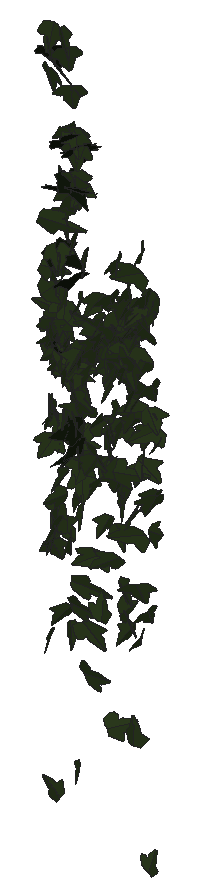
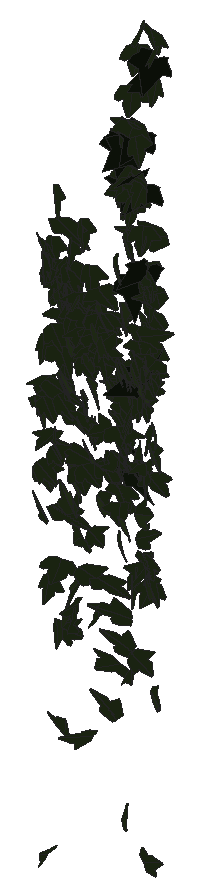
# SketchUp Ruby script. Lengths in millimetres.
U = 1.mm
M = Sketchup.active_model
def pt(a) = Geom::Point3d.new(a.map { |v| v * U })
def face(e, loops, mat)
  f = e.add_face(loops[0].map { |a| pt(a) })
  loops[1..].each { |l| e.add_face(l.map { |a| pt(a) }).erase! }
  f.material = f.back_material = mat if mat
  f
end
# faces: each face lists its corners as indices into pts; further lists are holes
def faces(e, pts, list, mat = nil) = list.each { |f| face(e, (f[0].is_a?(Array) ? f : [f]).map { |l| l.map { |i| pts[i] } }, mat) }
# xy, xz, yz: faces in a plane at the given z, y or x. An outline is a flat list of corners, or four numbers for a rectangle; further outlines are holes
def ring(l) = l.size == 4 ? [[l[0], l[1]], [l[2], l[1]], [l[2], l[3]], [l[0], l[3]]] : l.each_slice(2).to_a
def flat(e, list, mat, &to3) = list.each { |f| face(e, (f[0].is_a?(Array) ? f : [f]).map { |l| ring(l).map { |u, v| to3.(u, v) } }, mat) }
def xy(e, z, list, mat = nil) = flat(e, list, mat) { |x, y| [x, y, z] }
def xz(e, y, list, mat = nil) = flat(e, list, mat) { |x, z| [x, y, z] }
def yz(e, x, list, mat = nil) = flat(e, list, mat) { |y, z| [x, y, z] }
def lines(e, pts, list) = list.each { |a, b| e.add_line(pt(pts[a]), pt(pts[b])) }
# prism: a flat outline (further loops are holes) pulled along v
def prism(e, loops, v, mat = nil)
  f = face(e, loops, mat); d = Geom::Vector3d.new(v.map { |x| x * U })
  f.pushpull(f.normal.samedirection?(d) ? d.length : -d.length)
end
def box(e, o, s, mat = nil) = prism(e, [[o, [o[0] + s[0], o[1], o[2]], [o[0] + s[0], o[1] + s[1], o[2]], [o[0], o[1] + s[1], o[2]]]], [0, 0, s[2]], mat)
def at(x, y, z, deg = 0) = Geom::Transformation.translation(pt([x, y, z])) * Geom::Transformation.rotation(ORIGIN, Z_AXIS, deg.degrees)
def axes(o, x, y, z) = Geom::Transformation.new([*x, 0, *y, 0, *z, 0, *pt(o).to_a, 1])
def part(name) = M.definitions.add(name)
# library, detail: a bought-in or finely detailed component or shape, given as its bounding box
def library(name, o, s) = part(name).tap { |d| box(d.entities, o, s) }
def detail(e, o, s) = box(e.add_group.entities, o, s)
def put(e, d, t, mat = nil) = e.add_instance(d, t).tap { |i| i.material = mat if mat }
def group(e, t, mat = nil) = e.add_group.tap { |g| g.transformation = t; g.material = mat if mat }.entities
root = M.entities
M.materials.add("efeu1").color = [18, 25, 13]
M.materials.add("efeu2").color = [43, 57, 29]
c1 = part("ivyleaf_10")
p = [[0,12.8,-0.8],[-1.5,51.3,-10.9],[-4.9,51,-11.6],[-13.6,26.5,-7.3],[-13.2,15.9,-4.6],[-21.1,19.3,-7.2],
  [-29.5,16.3,-8.3],[-29.2,8.3,-6.2],[-19.7,-9.8,0.5],[-7.6,-13,4],[1,-12.2,5.8],[-0.4,51.1,-11.1],
  [-1.5,51.1,-10.9],[1,-12.4,5.9],[16.9,-12.4,3.5],[35.1,9.1,-5.1],[35,12.9,-6.1],[20.5,16.4,-4.9],
  [15.8,15,-3.8],[15.3,27.6,-7.1],[12.8,31.3,-7.8]]
faces(c1.entities,p,[[0,1,2,3,4,5,6,7,8,9,10],[11,12,0,13,14,15,16,17,18,19,20]],"efeu2")
c2 = part("ivyleaf_9")
p = [[39.1,54.8,31.7],[34.5,51.8,30.2],[-5.3,25.2,17.3],[-17.9,28.3,20.9],[-21.6,21.7,17],[-20.2,4.3,5.3],
  [-22.9,-0.3,2.5],[-17.1,-4,-0.6],[-2,-2.1,-1.2],[-0.7,-15.4,-10.1],[16.6,-22.3,-16.7],[21.1,-15.1,-12.5],
  [32.7,-10.7,-11],[46.1,-1.8,-6.6],[30.8,11.2,3.8]]
faces(c2.entities,p,[[0,1,2,3,4,5,6,7,8,9,10,11,12,13,14]],"efeu1")
put(root,c1,axes([788.1,1030.8,1427.8],[-0.8216,0.31601,0.08048],[-0.10582,0.00442,-0.74318],[-0.38351,-0.67822,0.03266]))
put(root,c1,axes([783.8,1037.2,366.4],[0.35503,-0.51907,0.28916],[0.17558,-0.25081,-0.59507],[0.70331,0.32464,0.00259]))
put(root,c1,axes([799.3,1035.4,70.7],[0.41211,-0.03589,0.60831],[-0.74004,0.04654,0.33959],[-0.07091,-0.69425,-0.00868]))
put(root,c1,axes([791.1,1037.6,927.4],[-0.31775,-0.66613,-0.05139],[0.00589,0.0522,-0.68667],[1.27154,-0.1667,-0.00966]))
put(root,c1,axes([800.6,1033.4,982.4],[0.2874,0.16747,0.66778],[-0.64392,-0.40925,0.28883],[0.5393,-0.57788,-0.01102]))
put(root,c2,axes([787.2,1031.5,1468.6],[0.6978,0.49681,-0.19291],[-0.15856,-0.14442,-0.75725],[-0.63057,0.58609,-0.02307]))
put(root,c1,axes([791.7,1032.9,898],[0.77102,0.08245,0.22157],[-0.26965,-0.01835,0.63726],[0.10235,-0.66944,0.00982]))
put(root,c1,axes([778.7,1041.7,950.2],[0.68596,0.18794,0.34559],[0.39955,0.11033,-0.59284],[-0.26587,0.65069,0.00071]))
put(root,c1,axes([799.9,1015.8,799.9],[0.1243,-0.11012,0.73702],[-0.66756,0.49393,0.14944],[-0.61718,-0.55643,-0.0132]))
put(root,c1,axes([792.3,1029.1,785.9],[0.2141,-0.65009,-0.01518],[0.00013,0.01541,-0.65975],[1.23759,0.11246,0.00269]))
put(root,c1,axes([793.1,1027.7,737.6],[0.73244,0.27951,-0.31616],[-0.34633,-0.13931,-0.66221],[-0.38094,0.66407,-0.00585]))
put(root,c1,axes([788.2,1029.7,1483.2],[-0.28744,0.74297,-0.0561],[0.00406,-0.05779,-0.7793],[-0.909,-0.2352,0.01426]))
put(root,c1,axes([797.4,1029.2,926.8],[0.31491,-0.02662,0.66088],[-0.48842,0.55843,0.17886],[-0.64233,-0.43767,0.18801]))
put(root,c1,axes([793.6,1033.7,556],[0.21115,-0.73707,0.09646],[-0.00653,-0.10027,-0.75661],[0.90687,0.17089,-0.02791]))
put(root,c1,axes([792.8,1042.4,897.2],[-0.01529,0.02833,0.67814],[0.09057,-0.67413,0.02954],[0.82309,0.07471,0.00935]))
put(root,c1,axes([793.5,1044.9,604.9],[0.83447,-0.2207,-0.05303],[-0.05883,0.02324,-0.71868],[0.27059,0.68565,0.00729]))
put(root,c1,axes([780.6,1028.3,1011.1],[0.68309,-0.13537,-0.48508],[0.56698,-0.14057,0.57566],[-0.2367,-0.72735,-0.02098]))
put(root,c1,axes([797.1,1043.7,878.8],[-0.07619,-0.6591,-0.00693],[0.00134,0.00686,-0.66205],[0.80415,-0.06246,0.00045]))
put(root,c1,axes([794.2,1036.8,564.8],[0.47786,-0.63117,0.09926],[0.07896,-0.07664,-0.74269],[0.77548,0.39673,0.01446]))
put(root,c1,axes([799.2,1028.6,591.4],[-0.32506,0.49635,0.38567],[-0.27259,0.31674,-0.562],[-0.71677,-0.34556,0.03883]))
put(root,c1,axes([793.7,1045.7,768.5],[0.39639,0.56977,-0.20295],[-0.12608,-0.19187,-0.60663],[-1.1442,0.21853,-0.00346]))
put(root,c1,axes([792.2,1027.3,1511],[0.91653,-0.22701,0.09119],[0.10411,-0.03284,-0.78478],[0.27971,0.75606,-0.00671]))
put(root,c1,axes([783.4,1027.2,1061.1],[-0.1807,-0.20858,-0.64289],[0.74252,0.24504,-0.21972],[0.35857,-0.61253,0.13101]))
put(root,c2,axes([801.5,1036.1,912.9],[0.18122,-0.67532,0.32709],[-0.03577,0.32796,0.69043],[-0.91475,-0.14661,0.0378]))
put(root,c1,axes([798.6,1023.2,951.7],[-0.19091,0.66075,0.24701],[-0.20959,0.2097,-0.66978],[-0.83469,-0.20378,0.11169]))
put(root,c1,axes([798.3,1031.9,935.2],[0.07288,-0.62882,-0.29154],[0.11181,0.29388,-0.62614],[1.31439,0.00987,0.06943]))
put(root,c1,axes([808.1,1033.5,1069.4],[0.29042,-0.0913,-0.66321],[-0.45833,0.5644,-0.21254],[0.67603,0.42187,0.14082]))
put(root,c1,axes([804.1,1038.4,939.6],[0.34517,-0.6149,-0.26073],[-0.05992,0.262,-0.6398],[1.26972,0.17952,0.04068]))
put(root,c1,axes([798.6,1025.5,544.7],[-0.59363,-0.39577,-0.2622],[0.25431,0.15923,-0.62717],[0.52037,-0.5293,0.00739]))
put(root,c1,axes([803.6,1039.9,1166.3],[-0.57926,-0.51111,-0.06286],[0.0462,0.05062,-0.69758],[0.62655,-0.47626,-0.00668]))
put(root,c1,axes([803.7,1033,743.6],[0.44885,-0.47733,-0.38288],[-0.02835,0.40573,-0.515],[1.16425,0.1939,0.13507]))
put(root,c1,axes([801.6,1021.3,1048.5],[0.70382,-0.53867,-0.29794],[0.06531,0.36507,-0.61744],[1.16973,0.30373,0.21374]))
put(root,c1,axes([801.7,1024.1,960.1],[-0.89528,-0.26816,-0.13173],[0.17561,-0.01121,-0.77906],[0.3194,-0.74548,0.0591]))
put(root,c1,axes([806,1032.1,893],[-0.53685,0.56978,0.24643],[-0.25649,0.14743,-0.71629],[-0.7126,-0.48231,0.07216]))
put(root,c1,axes([805.1,1018.8,807.1],[-0.51279,0.56779,0.11249],[-0.09933,0.07964,-0.70621],[-0.69914,-0.42776,0.01783]))
put(root,c1,axes([806.4,1037.6,632.5],[-0.02983,-0.02156,0.66723],[-0.01438,-0.66756,-0.022],[0.81432,-0.01258,0.02405]))
put(root,c1,axes([805.3,1025.6,1084],[0.74042,-0.59205,-0.15393],[0.02348,0.18998,-0.69951],[1.16401,0.37276,0.11203]))
put(root,c1,axes([796.1,1041,881.8],[0.26766,-0.51968,-0.31436],[0.36513,-0.19834,0.53676],[-0.64477,-0.32805,0.17347]))
put(root,c1,axes([809.4,1031.6,585.8],[0.02991,0.54049,-0.53466],[-0.31756,-0.49664,-0.51399],[-0.87145,0.19953,0.16895]))
put(root,c1,axes([808.2,1043.6,792.7],[-0.25794,0.57627,-0.25871],[-0.14917,-0.2779,-0.57795],[-1.19293,-0.08985,0.12821]))
put(root,c1,axes([813.5,1034.4,875.5],[-0.75172,0.38055,0.21329],[-0.24032,0.08664,-0.72364],[-0.47488,-0.64625,0.02858]))
put(root,c1,axes([804.4,1025.5,1100.7],[0.53358,0.59441,0.03481],[0.02364,0.02896,-0.73798],[-0.72604,0.43779,0.00155]))
put(root,c1,axes([815.2,1040.2,422.2],[-0.2053,-0.57396,0.34459],[-0.10385,-0.34034,-0.58396],[1.26988,-0.12063,0.00795]))
put(root,c1,axes([811.7,1045,1320.9],[-0.14471,-0.72719,-0.02028],[0.01042,0.01915,-0.73678],[0.88745,-0.1188,0.00535]))
put(root,c2,axes([795.6,1037.4,1436.5],[0.77726,-0.42672,0.06495],[0.05255,-0.05237,-0.76655],[0.52396,0.63826,-0.01947]))
put(root,c1,axes([807.4,1040.3,968.4],[0.79768,0.23933,-0.04503],[-0.05019,-0.01861,-0.69625],[-0.29283,0.65512,-0.00333]))
put(root,c1,axes([810,1039.5,1237.5],[-0.75298,0.34973,-0.07002],[0.06708,-0.04498,-0.70929],[-0.42993,-0.61953,0.01197]))
put(root,c1,axes([805.1,1036.6,578.9],[0.34309,0.56152,0.42564],[0.12442,0.42103,-0.62281],[-0.85058,0.28808,0.08059]))
put(root,c1,axes([809.7,1038.4,672.6],[0.17239,-0.27183,0.6442],[0.33118,-0.62038,-0.28625],[1.28885,0.19577,-0.01261]))
put(root,c1,axes([812.4,1033.4,1018],[0.67283,-0.43188,0.01125],[0.01059,-0.00716,-0.70048],[0.52696,0.55157,-0.00028]))
put(root,c2,axes([804.3,1028.5,1101.2],[0.05905,-0.29496,-0.71405],[0.10041,0.71335,-0.28909],[0.93718,-0.05785,0.07596]))
put(root,c1,axes([807.8,1035.5,1154.9],[-0.49133,0.44585,-0.38218],[0.28029,-0.30685,-0.60007],[-0.65932,-0.4627,0.0297]))
put(root,c1,axes([811.9,1043.3,944.4],[0.77211,-0.28069,0.04328],[0.04739,-0.01918,-0.69233],[0.34323,0.63407,-0.00178]))
put(root,c1,axes([814.9,1047.6,927],[0.26366,-0.6216,0.13768],[0.05873,-0.12903,-0.65809],[0.77451,0.22139,0.00303]))
put(root,c1,axes([811.5,1035.4,992.2],[0.78518,0.26762,0.03048],[0.03439,0.0116,-0.69701],[-0.3268,0.6442,-0.00012]))
put(root,c1,axes([816.6,1018.4,900.3],[0.22008,0.15461,-0.73651],[0.11954,0.74611,0.18062],[0.91032,-0.13535,0.15434]))
put(root,c1,axes([820.6,1032.1,767.5],[0.42794,-0.56327,-0.2545],[-0.04803,0.26223,-0.60266],[1.17538,0.21579,0.06803]))
put(root,c1,axes([820.2,1033.2,1473.6],[-0.62749,-0.57058,-0.10471],[0.10493,0.06339,-0.76789],[0.69991,-0.52105,0.02124]))
put(root,c1,axes([793.1,1019.4,1156],[-0.26864,-0.01399,-0.72946],[1.38215,0.06866,-0.14184],[0.13336,-0.73981,0.00063]))
put(root,c1,axes([819.9,1041.6,553.1],[0.284,-0.67396,-0.27143],[0.02977,0.29211,-0.70439],[0.88591,0.20623,0.11068]))
put(root,c1,axes([817.2,1027.9,1508],[-0.27935,0.74611,-0.10082],[0.05762,-0.09094,-0.78024],[-0.91672,-0.23308,-0.01832]))
put(root,c1,axes([825.9,1038.2,1402.2],[-0.72465,-0.46268,-0.06511],[0.0655,0.03703,-0.7529],[0.56625,-0.59638,0.00376]))
put(root,c2,axes([809.2,1032.3,898.4],[0.83233,0.09053,0.33278],[0.38329,0.14109,-0.68248],[-0.17354,0.74584,0.08871]))
put(root,c1,axes([820.3,1045.1,869.1],[1.19887,0.22319,0.03324],[0.05223,0.02207,-0.66819],[-0.42627,0.63041,0.01162]))
put(root,c1,axes([829.5,1028.5,889],[0.22544,-0.73184,0.13191],[0.04657,-0.12641,-0.75478],[0.90603,0.1886,0.00598]))
put(root,c1,axes([829.4,1032.1,1204.4],[-0.09943,-0.71279,-0.30144],[0.12916,0.28999,-0.71433],[0.93529,-0.11583,0.0666]))
put(root,c1,axes([829.2,1040.7,829.3],[-0.48196,0.62803,0.05802],[-0.04399,0.04586,-0.74193],[-0.7682,-0.39665,0.00609]))
put(root,c2,axes([826.5,1013.4,1318.6],[0.60636,0.62737,0.15242],[0.11435,0.12019,-0.80039],[-0.77931,0.50578,0.00114]))
put(root,c1,axes([829.2,1037.1,848.5],[-0.38653,0.67633,0.09582],[-0.03231,0.09339,-0.7467],[-0.83274,-0.31755,-0.01551]))
put(root,c2,axes([836.5,1021.4,1058],[0.12899,0.77979,-0.05082],[-0.04045,-0.04676,-0.78647],[-0.9525,0.10759,0.02652]))
put(root,c2,axes([827.6,1012.6,1228.8],[1.09201,0.49687,0.00466],[-0.18424,0.11876,-0.7434],[-0.92757,0.56137,0.15315]))
put(root,c2,axes([843.3,1024.8,732.6],[-0.56978,0.62886,-0.13687],[-0.02843,-0.18552,-0.77289],[-0.78466,-0.44993,0.12739]))
put(root,c1,axes([828.7,1035.6,394.8],[-0.10488,0.66245,-0.25128],[0.01968,-0.25123,-0.66783],[-0.86415,-0.08612,0.01529]))
put(root,c1,axes([829,1030.1,1216.6],[-0.57705,-0.55815,-0.2835],[0.31687,0.14833,-0.72538],[0.69492,-0.53112,0.09534]))
put(root,c1,axes([836,1039,899.5],[0.28093,-0.59692,-0.29532],[-0.08494,0.29294,-0.61442],[1.26464,0.15227,0.02434]))
put(root,c2,axes([847.7,1025.3,776],[-0.81069,0.36511,0.18835],[-0.19173,0.10503,-0.75803],[-0.46309,-0.68265,-0.01589]))
put(root,c1,axes([841.5,1029.1,779.7],[0.25086,-0.1414,-0.71854],[-0.22369,0.71262,-0.1927],[0.86498,0.2253,0.15855]))
put(root,c1,axes([835.1,1026.1,1331.6],[-0.87588,-0.27757,-0.18304],[0.20906,0.06437,-0.76972],[0.34761,-0.7381,0.0017]))
put(root,c1,axes([844.7,1045.2,806.6],[-0.87106,-0.42721,0.18591],[-0.17432,-0.17301,-0.62307],[0.8694,-0.46271,0.06133]))
put(root,c1,axes([836.3,1037.9,1137.4],[0.37676,-0.66256,0.17446],[0.10123,-0.15379,-0.73093],[0.82972,0.31962,0.00995]))
put(root,c2,axes([835.5,1029.5,1296.2],[0.64762,0.47884,0.32201],[0.12075,0.35551,-0.6918],[-0.69356,0.50901,0.18024]))
put(root,c1,axes([843.6,1031.9,912.2],[-0.35777,-0.56059,0.37592],[0.04576,-0.42277,-0.6012],[0.82219,-0.22041,0.19704]))
put(root,c1,axes([842.1,1038.5,1226.6],[0.82885,0.32894,-0.15258],[-0.22383,0.03232,-0.74722],[-0.38158,0.69556,0.10688]))
put(root,c2,axes([831.6,1025.9,1246.1],[0.24476,-0.68834,-0.34335],[0.0045,0.35569,-0.71093],[0.93844,0.17782,0.09296]))
put(root,c1,axes([832,1044.2,637.7],[-0.05394,-0.28985,-0.63625],[0.4019,-0.57095,0.23721],[-0.75236,-0.28422,0.17233]))
put(root,c1,axes([840.7,1042.5,920.6],[0.70286,-0.4529,0.05393],[0.03657,-0.0491,-0.73255],[0.55524,0.57655,-0.02002]))
put(root,c1,axes([845.5,1039.6,777.7],[0.55897,-0.5521,-0.18873],[-0.08514,0.18936,-0.62357],[1.1072,0.2933,0.04733]))
put(root,c1,axes([846.7,1034,1014.4],[0.22774,-0.64549,-0.27399],[-0.04686,0.27391,-0.65606],[1.33377,0.11984,0.02373]))
put(root,c1,axes([842.4,1033.8,1236.7],[0.07605,0.72342,0.24404],[-0.1281,0.25065,-0.7162],[-0.92259,0.02483,0.11956]))
put(root,c1,axes([845.9,1026.5,1303.9],[-0.95552,-0.11615,0.01117],[0.01741,-0.17059,-0.77313],[0.14129,-0.76449,0.17082]))
put(root,c1,axes([834.2,1023.7,1237.5],[0.84937,0.17225,0.32875],[0.29571,0.31821,-0.68003],[-0.3429,0.70109,0.22788]))
put(root,c1,axes([840.1,1025.7,1249.9],[-0.76524,-0.38994,-0.28867],[0.36551,0.0598,-0.73177],[0.46556,-0.68789,0.10002]))
put(root,c2,axes([849.9,1029.8,757.2],[-0.81763,0.21596,-0.35153],[0.40023,-0.12767,-0.70388],[-0.30521,-0.74594,0.0187]))
put(root,c1,axes([837,1053.4,752.1],[0.41766,-0.40903,0.4743],[0.45844,-0.29829,-0.52848],[0.61129,0.50317,0.07227]))
put(root,c1,axes([837.5,1050.7,613.6],[0.44688,-0.32575,0.49459],[0.426,-0.35092,-0.48973],[0.58357,0.50562,-0.02125]))
put(root,c1,axes([845.7,1039.7,704.8],[0.91379,0.04342,-0.11895],[-0.14633,0.01445,-0.74997],[-0.04954,0.75826,0.02111]))
put(root,c1,axes([825.4,1023.7,892.5],[-0.06992,-0.2027,-0.70056],[1.18354,0.35774,-0.13612],[0.72511,-0.60346,0.15463]))
put(root,c1,axes([835.9,1039.3,744.1],[1.04002,0.2779,-0.31031],[0.49606,0.17116,0.61229],[0.61842,-0.60466,0.03071]))
put(root,c2,axes([849.3,1025.4,1303],[0.39684,0.71981,-0.02665],[-0.01813,-0.02253,-0.78989],[-0.87859,0.32559,0.00426]))
put(root,c1,axes([840.2,1038.6,132.5],[0.08906,-0.17636,0.61055],[0.47215,-0.47513,-0.18352],[0.61498,0.39032,0.05248]))
put(root,c1,axes([850.6,1039.4,918],[0.35486,-0.70755,-0.02213],[-0.00839,0.0211,-0.76501],[0.8636,0.29094,0.00166]))
put(root,c1,axes([845.6,1041.1,675.5],[0.65263,0.52861,0.02722],[0.02376,0.01902,-0.75206],[-0.64532,0.5353,-0.00016]))
put(root,c1,axes([843.2,1023.4,1330.3],[0.90217,0.07386,0.24658],[0.29125,0.08374,-0.741],[-0.11745,0.775,0.05657]))
put(root,c1,axes([845.9,1051.4,1094.6],[0.43331,-0.45589,0.46148],[0.37791,-0.34308,-0.57732],[0.69535,0.47055,0.02618]))
put(root,c1,axes([837.4,1037.9,823.4],[-0.07041,0.01632,-0.74835],[0.76134,-0.41342,-0.05714],[-0.50428,-0.62645,0.01822]))
put(root,c1,axes([849.6,1036.8,719.5],[-0.4111,0.46787,0.50899],[0.36967,-0.409,0.57656],[0.75812,0.45314,-0.00513]))
put(root,c1,axes([837.8,1053.3,845.3],[0.28015,-0.15426,0.62818],[0.91906,-0.40242,-0.21198],[0.81907,0.50431,0.023]))
put(root,c1,axes([835.3,1038.8,433.2],[-0.2924,-0.08574,0.63617],[1.21476,-0.09001,0.14201],[0.12999,0.64823,0.10386]))
put(root,c1,axes([859.3,1047.1,885.7],[0.12154,-0.62602,0.23795],[0.11007,-0.23298,-0.62847],[1.26984,0.08011,0.0317]))
put(root,c1,axes([873.5,1045.8,538.5],[0.85734,0.13049,-0.44841],[-0.81592,-0.13156,-0.46896],[-0.35252,0.62184,-0.00512]))
put(root,c1,axes([875.7,1041.5,949.6],[-0.16089,-0.66887,0.15832],[-0.02121,-0.15816,-0.67413],[1.30799,-0.08484,0.00854]))
put(root,c1,axes([847.4,1032.5,481.8],[0.07239,-0.025,0.6654],[1.21024,0.19907,-0.02887],[-0.37592,0.63606,0.03519]))
put(root,c1,axes([875.4,1041.3,926.7],[-0.40725,-0.64863,-0.10876],[0.06436,0.10337,-0.68301],[1.25004,-0.21664,-0.00027]))
put(root,c1,axes([896.2,1027.6,978.2],[-0.69899,-0.00816,-0.60624],[-1.15386,-0.00048,0.3673],[-0.00883,0.70881,-0.00673]))
put(root,c1,axes([879.7,1032,729.1],[-0.59741,-0.52713,0.19046],[-0.08935,-0.1928,-0.61098],[1.06296,-0.31247,0.05569]))
put(root,c1,axes([876.1,1047.8,678.6],[0.18482,-0.57688,0.26469],[0.04381,-0.2644,-0.58468],[1.20718,0.09792,-0.01931]))
put(root,c1,axes([854.4,1041.9,399.1],[0.91037,0.05986,0.45963],[0.87245,0.03668,-0.48184],[-0.13059,0.66236,-0.01486]))
put(root,c1,axes([889.1,1045.7,940.1],[-1.09676,-0.12874,-0.3437],[-0.64444,-0.06035,0.59033],[-0.26948,0.66826,-0.0129]))
put(root,c1,axes([860.3,1040.9,311.2],[-0.60281,0.08852,0.62038],[1.14404,-0.15355,0.32881],[0.33709,0.67943,-0.00652]))
put(root,c1,axes([887.3,1034.2,983],[-0.98341,-0.45117,0.15095],[-0.10156,-0.16648,-0.68027],[0.89974,-0.51192,0.0882]))
put(root,c1,axes([888.6,1034.8,1031.9],[0.64538,0.52783,-0.30852],[-0.5616,-0.16768,-0.61122],[-1.01909,0.42668,0.14145]))
put(root,c1,axes([860,1040.3,734],[0.35495,-0.17478,0.66487],[1.20554,-0.22402,-0.23657],[0.50844,0.65318,0.09677]))
put(root,c1,axes([883.2,1030.9,791.3],[0.12924,-0.15701,0.70428],[-0.21915,0.69597,0.16626],[-1.35569,-0.12747,0.04027]))
put(root,c1,axes([888.4,1037,993.2],[0.53302,-0.6353,0.11245],[0.05885,-0.10923,-0.69412],[1.22649,0.28134,-0.01556]))
put(root,c1,axes([893.6,1038.6,966.9],[0.02212,-0.69001,0.11879],[-0.01225,-0.11891,-0.69006],[1.33249,0.01036,-0.00832]))
put(root,c1,axes([893.3,1044.5,928.1],[-1.28448,-0.02529,-0.01054],[0.02864,-0.1251,-0.66361],[0.04357,-0.66329,0.12556]))
put(root,c1,axes([906.7,1048,543.4],[-0.51504,-0.33223,0.47396],[-0.50877,-0.39232,-0.42764],[0.97706,-0.37942,0.02716]))
put(root,c1,axes([894,1047.2,613.4],[-0.18746,-0.50468,0.37459],[0.15604,-0.38624,-0.49882],[1.18596,-0.02895,0.12484]))
put(root,c1,axes([903.9,1051.4,723.2],[-0.56451,-0.47972,0.32499],[-0.09283,-0.34313,-0.55101],[1.09887,-0.27543,0.12041]))
put(root,c1,axes([901.4,1045.6,917.7],[-0.00405,-0.4887,0.47237],[-0.01283,-0.47234,-0.4887],[1.29351,-0.00621,-0.00337]))
put(root,c1,axes([903.8,1039.1,865.9],[0.40105,-0.62079,-0.12843],[-0.08641,0.12022,-0.65556],[1.2034,0.21552,-0.00427]))
put(root,c1,axes([907.2,1013.4,452.9],[0.2344,0.56395,-0.45611],[0.05779,0.45822,0.57476],[1.3792,-0.11504,0.05343]))
put(root,c1,axes([903.5,1044.6,933.5],[0.31124,0.59311,-0.30164],[-0.1304,-0.29395,-0.61515],[-1.25967,0.17698,-0.01085]))
put(root,c1,axes([906.5,1040.3,985.2],[-1.1725,-0.2928,-0.13396],[0.23991,0.0468,-0.68201],[0.56389,-0.62872,0.01162]))
put(root,c1,axes([910.9,1042.4,934.3],[-1.14439,0.30957,-0.03744],[0.04898,-0.03178,-0.67611],[-0.59143,-0.60162,0.01645]))
put(root,c1,axes([914.3,1041.9,903.7],[-0.36258,-0.60733,0.2591],[0.06491,-0.27836,-0.6274],[1.25498,-0.16107,0.10731]))
put(root,c1,axes([898,1048.3,788.9],[0.11349,-0.17735,0.64298],[0.85255,-0.46763,-0.17053],[0.94051,0.4453,0.07699]))
put(root,c1,axes([914.6,1031.3,916.3],[0.75619,-0.54573,0.04905],[0.04312,-0.04417,-0.675],[1.04193,0.3979,-0.00766]))
put(root,c1,axes([917.9,1024,1050.7],[-0.29529,-0.68174,-0.17317],[0.07075,0.16914,-0.69917],[1.33683,-0.15954,-0.00125]))
put(root,c1,axes([903.3,1035.3,778.7],[0.28832,-0.37032,0.60658],[0.8345,-0.43939,-0.37776],[1.06446,0.44477,0.13185]))
put(root,c1,axes([908.1,1028,722.5],[0.61433,-0.50679,-0.23509],[0.27894,-0.18518,0.60043],[-1.02601,-0.35379,0.02248]))
put(root,c1,axes([921.8,1035.1,836.5],[0.42168,-0.58135,-0.21067],[-0.01857,0.22047,-0.61866],[1.17668,0.21182,0.06573]))
put(root,c1,axes([925.3,1041.6,707.2],[-0.49586,-0.59721,0.03733],[-0.02357,-0.03533,-0.65156],[1.13858,-0.26082,0.00277]))
put(root,c1,axes([934,1042.7,801.5],[0.94846,-0.14972,-0.43723],[-0.80068,0.11922,-0.52033],[0.36411,0.65216,-0.00526]))
put(root,c1,axes([926,1027.5,982.6],[-1.32605,-0.05569,0.03148],[-0.0601,-0.00006,-0.69896],[0.10588,-0.69746,-0.00245]))
put(root,c1,axes([918.6,1042.7,956.9],[0.36084,0.66435,0.01771],[-0.0173,0.021,-0.69073],[-1.26473,0.18926,0.0145]))
put(root,c1,axes([922.3,1036.5,1010],[0.61237,0.59895,0.15796],[-0.15631,0.21767,-0.6581],[-1.16849,0.28477,0.17081]))
put(root,c1,axes([924.6,1030,989.6],[-0.67269,0.60457,-0.05381],[0.03018,-0.05305,-0.70019],[-1.15478,-0.35356,0.01305]))
put(root,c1,axes([949.9,1020.6,950.5],[-0.82678,0.15384,0.56092],[-1.06595,0.07816,-0.4552],[-0.29853,-0.70515,0.07191]))
put(root,c1,axes([914.3,1049.8,600.9],[0.75369,-0.27152,0.42386],[0.70884,-0.20474,-0.47913],[0.64445,0.54274,0.0313]))
put(root,c1,axes([920,1050.9,676.9],[-0.07565,-0.16741,-0.62246],[0.30842,-0.6062,0.15269],[-1.18736,-0.1468,0.07932]))
put(root,c1,axes([928.8,1035.4,983.9],[1.32455,-0.00157,-0.05339],[-0.10129,0.03876,-0.69489],[0.00862,0.69693,0.03853]))
put(root,c1,axes([932.7,1022.2,1124.7],[0.01085,-0.70385,-0.21452],[0.11172,0.21428,-0.7015],[1.39594,-0.01168,0.05781]))
put(root,c1,axes([926.4,1037.9,798.9],[0.2765,-0.35829,0.54775],[0.46672,-0.49042,-0.38583],[1.15496,0.28396,0.02478]))
put(root,c1,axes([925.8,1050.3,658.2],[0.18958,-0.45209,0.44859],[0.50777,-0.38267,-0.44489],[1.10063,0.25441,0.12798]))
put(root,c1,axes([921.3,1027,242.7],[0.39186,-0.03249,-0.68031],[0.75784,0.58234,0.0927],[1.05162,-0.40755,0.18669]))
put(root,c1,axes([934,1039.2,505.2],[-0.45609,0.67302,0.18709],[-0.11813,0.17649,-0.71442],[-1.32421,-0.24755,-0.0007]))
put(root,c1,axes([939.1,1029.7,943.5],[-1.22303,0.23144,0.02187],[-0.0527,-0.01237,-0.6827],[-0.43928,-0.64287,0.02101]))
put(root,c1,axes([936.5,1040.5,980.4],[-0.52202,-0.55238,-0.32377],[0.24409,0.29768,-0.61654],[1.19387,-0.30239,-0.01551]))
put(root,c1,axes([930.8,1028.2,919.6],[-1.07083,0.15192,-0.34681],[0.61009,-0.13943,-0.58114],[-0.38347,-0.64607,0.04387]))
put(root,c1,axes([942.9,1045.1,427],[-0.07933,-0.39071,0.54145],[0.17347,-0.54075,-0.38319],[1.25887,0.04989,0.08692]))
put(root,c1,axes([940.2,1030.9,464.8],[0.12395,0.02379,-0.69063],[0.30611,0.67412,0.03839],[1.27907,-0.16364,0.05774]))
put(root,c1,axes([949.4,1031.3,1047.3],[-0.37527,-0.67574,0.13557],[-0.03589,-0.13567,-0.70365],[1.31121,-0.19711,0.01954]))
put(root,c1,axes([946.2,1036.8,926.8],[0.19341,-0.64984,0.18183],[0.0728,-0.17804,-0.65766],[1.28221,0.10813,0.00991]))
put(root,c1,axes([951.7,1039,431.7],[-0.82118,0.46856,-0.05166],[-0.07774,0.0326,0.63691],[0.89379,0.43333,0.00794]))
put(root,c1,axes([946.5,1050,871.7],[0.39441,-0.64225,0.25846],[0.14871,-0.24636,-0.67486],[1.30918,0.22147,-0.00121]))
put(root,c1,axes([952,1049.8,826.6],[-0.27091,-0.59627,0.23499],[-0.05298,-0.23473,-0.61249],[1.21862,-0.14276,0.02561]))
put(root,c1,axes([948.2,1037.8,1000.8],[1.10529,-0.39263,-0.0221],[-0.05306,-0.00178,-0.70081],[0.74655,0.58117,-0.01708]))
put(root,c1,axes([953.7,1035.5,1040.5],[0.9712,-0.4078,-0.26684],[-0.28532,0.23627,-0.64778],[0.88254,0.52515,0.08422]))
put(root,c1,axes([941.6,1038.1,1012],[-0.68204,0.49503,-0.3433],[0.3961,-0.27312,-0.61108],[-1.07592,-0.41435,-0.00735]))
put(root,c1,axes([953.1,1025.6,694.8],[0.49232,-0.58764,-0.06946],[-0.04288,0.06597,-0.64203],[1.12537,0.25959,0.00592]))
put(root,c1,axes([973.3,1046.9,844.7],[-0.65924,0.01985,0.57524],[-1.03092,-0.23825,-0.31795],[0.3704,-0.62778,0.13886]))
put(root,c1,axes([966.8,1037.4,899.2],[-1.09711,0.16029,0.35396],[-0.66251,0.06832,-0.59786],[-0.32857,-0.67299,0.02361]))
put(root,c1,axes([954.9,1047.2,860.7],[0.41676,-0.62826,0.04849],[0.00363,-0.05068,-0.66517],[1.19926,0.21848,-0.01484]))
put(root,c1,axes([957.5,1030.3,1005],[0.15149,-0.68003,-0.18076],[-0.02412,0.1805,-0.68462],[1.33895,0.08019,0.00812]))
put(root,c1,axes([956.9,1037.7,1008.6],[0.39541,-0.62379,-0.25004],[-0.00324,0.26123,-0.65311],[1.27902,0.1935,0.07565]))
put(root,c1,axes([971.9,1028,620.2],[0.78769,0.00667,-0.5406],[-1.02884,0.01472,-0.41369],[0.01453,0.68068,0.01424]))
put(root,c1,axes([957.4,1018.6,1081.5],[0.08554,-0.62259,-0.38285],[0.13569,0.38548,-0.61849],[1.38438,0.00069,0.08428]))
put(root,c1,axes([929.9,1027.4,725.6],[0.42614,-0.11575,-0.69846],[1.30151,-0.15429,0.24479],[-0.34882,-0.71706,0.06008]))
put(root,c1,axes([971.9,1021.7,1114.2],[0.98692,-0.09953,-0.48932],[-0.8657,0.19687,-0.52209],[0.39206,0.68525,0.07893]))
put(root,c1,axes([952.4,1033.3,636.4],[0.26904,-0.72803,-0.09826],[0.06264,-0.09369,0.74149],[-1.39674,-0.14444,0.01433]))
put(root,c1,axes([959,1028.7,964.1],[1.20497,0.2487,-0.1297],[-0.27029,0.00812,-0.67771],[-0.46033,0.64623,0.05843]))
put(root,c1,axes([964.9,1051.9,734.7],[-0.28281,-0.54278,0.31521],[0.19029,-0.34026,-0.53878],[1.17933,-0.07526,0.16252]))
put(root,c1,axes([969.7,1028.9,998.7],[-0.53045,-0.62264,0.16039],[0.03681,-0.18285,-0.67622],[1.22313,-0.26452,0.08991]))
put(root,c1,axes([969,1031.1,1030],[0.05199,-0.69814,-0.03875],[0.0105,0.039,-0.69864],[1.33071,0.02697,0.00703]))
put(root,c1,axes([969.4,1025.9,235.9],[1.03246,-0.3464,0.26823],[-0.42826,0.14599,0.64365],[-0.71542,-0.5873,0.00179]))
put(root,c1,axes([971.5,1035.7,422.7],[-0.03908,-0.52228,-0.39569],[-0.01893,0.39609,-0.52228],[1.24691,-0.01035,-0.02033]))
put(root,c1,axes([954.8,1028.1,932.5],[0.97471,-0.28134,0.36102],[0.63682,-0.13951,-0.58339],[0.59434,0.61087,0.03303]))
put(root,c1,axes([965.5,1021.8,1045.2],[-0.08885,-0.43629,-0.5854],[0.36111,0.55919,-0.43189],[1.34179,-0.17938,0.07747]))
put(root,c1,axes([971.3,1031.8,1006],[-0.06974,-0.68496,-0.10572],[0.05761,0.10418,-0.6855],[1.31778,-0.0408,0.02437]))
put(root,c1,axes([974.4,1040.1,936.3],[-0.48904,-0.62563,0.16499],[0.00445,-0.17842,-0.67292],[1.23139,-0.24782,0.06796]))
put(root,c1,axes([969.3,1035.1,1028.1],[-0.81914,0.54258,-0.14674],[-0.01109,-0.18912,-0.68218],[-1.06968,-0.41354,0.11945]))
put(root,c1,axes([965.4,1036.4,1022.8],[0.09007,0.67843,0.19217],[0.02473,0.19173,-0.68008],[-1.34177,0.04907,0.00036]))
put(root,c1,axes([961.3,1053.7,749.3],[0.44995,-0.31715,0.55644],[0.64296,-0.44217,-0.39556],[1.0356,0.41232,0.00382]))
put(root,c1,axes([975.5,1026.5,523.7],[-0.90321,-0.39617,-0.18142],[0.26257,0.11783,-0.6182],[0.78662,-0.49421,-0.00196]))
put(root,c1,axes([991.5,1019.5,1016.8],[-1.05132,0.19619,0.39944],[-0.72839,0.11547,-0.58598],[-0.43219,-0.67183,0.01593]))
put(root,c1,axes([985.9,1034.2,1037.4],[-0.4267,-0.35256,0.57167],[-0.20358,-0.57624,-0.39733],[1.26196,-0.21217,0.1292]))
put(root,c1,axes([984.7,1047.8,810.5],[-0.39834,-0.60601,0.18091],[0.04112,-0.1973,-0.63591],[1.20295,-0.19393,0.08164]))
put(root,c1,axes([995,1043.3,815.7],[0.64903,0.2431,-0.52089],[-0.79609,-0.31049,-0.41875],[-0.7504,0.53965,-0.00628]))
put(root,c1,axes([987.3,1019.7,1163.5],[0.22335,-0.65889,-0.32619],[0.00974,0.33104,-0.66685],[1.39922,0.10287,0.05671]))
put(root,c1,axes([991.8,1048.9,696.1],[-0.14048,-0.60581,0.323],[-0.04623,-0.32235,-0.61015],[1.3058,-0.07659,0.01315]))
put(root,c1,axes([990.6,1024.3,1076.3],[-0.17806,-0.66841,-0.24276],[0.08435,0.2389,-0.67485],[1.35079,-0.10303,0.01014]))
put(root,c1,axes([982.5,1034.5,751.6],[0.31782,0.56416,0.32934],[0.17297,0.31656,-0.58835],[-1.23118,0.19011,0.00236]))
put(root,c1,axes([996,1041.6,690.4],[-0.38126,-0.65298,0.10318],[-0.04649,-0.10043,-0.683],[1.25732,-0.20172,0.00603]))
put(root,c1,axes([999,1029,1056.3],[0.27731,-0.58366,-0.38437],[-0.13117,0.37872,-0.60121],[1.32358,0.15982,0.02095]))
put(root,c1,axes([988.8,1042.3,848],[0.34717,0.63323,0.07754],[0.04191,0.07435,-0.65898],[-1.21344,0.18374,-0.00057]))
put(root,c1,axes([997.1,1023.8,485],[-0.30397,-0.5508,-0.34731],[0.15264,0.33824,-0.5733],[1.22984,-0.17812,-0.01469]))
put(root,c1,axes([996.2,1037.7,1050.7],[0.62272,-0.56485,-0.26269],[0.06851,0.31337,-0.62898],[1.1836,0.27904,0.17461]))
put(root,c1,axes([984.9,1054.4,619.1],[0.19962,-0.29457,-0.5666],[0.50589,-0.50195,0.31016],[-1.10509,-0.28299,0.03964]))
put(root,c1,axes([999.2,1032.9,906.8],[-0.16491,-0.63688,-0.23448],[0.20325,0.22065,-0.63877],[1.27557,-0.1175,0.07147]))
put(root,c1,axes([1004.4,1042.6,801.5],[0.21462,-0.61552,-0.23177],[-0.12797,0.22313,-0.62529],[1.24519,0.12902,-0.02431]))
put(root,c1,axes([1001.6,1022.1,8.2],[0.26423,0.29865,-0.54476],[0.11256,0.54931,0.31622],[1.17699,-0.11958,0.09206]))
put(root,c1,axes([1003.3,1032,1074.3],[0.87405,-0.54338,-0.06754],[0.0047,0.09021,-0.70894],[1.04211,0.45534,0.05985]))
